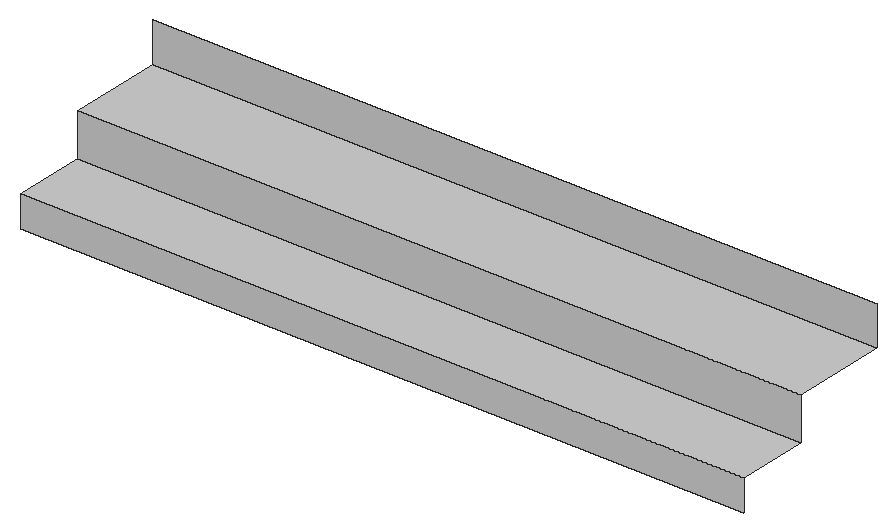
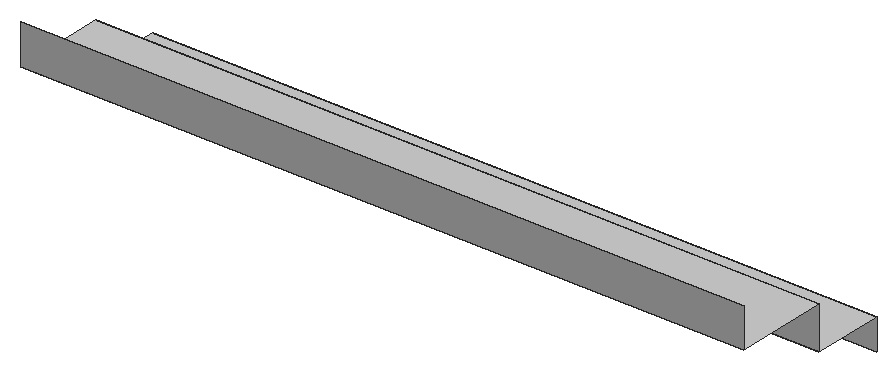
# SketchUp Ruby script. Lengths in inches.
U = 1.inch
M = Sketchup.active_model
def pt(a) = Geom::Point3d.new(a.map { |v| v * U })
def face(e, loops, mat)
  f = e.add_face(loops[0].map { |a| pt(a) })
  loops[1..].each { |l| e.add_face(l.map { |a| pt(a) }).erase! }
  f.material = f.back_material = mat if mat
  f
end
# faces: each face lists its corners as indices into pts; further lists are holes
def faces(e, pts, list, mat = nil) = list.each { |f| face(e, (f[0].is_a?(Array) ? f : [f]).map { |l| l.map { |i| pts[i] } }, mat) }
# xy, xz, yz: faces in a plane at the given z, y or x. An outline is a flat list of corners, or four numbers for a rectangle; further outlines are holes
def ring(l) = l.size == 4 ? [[l[0], l[1]], [l[2], l[1]], [l[2], l[3]], [l[0], l[3]]] : l.each_slice(2).to_a
def flat(e, list, mat, &to3) = list.each { |f| face(e, (f[0].is_a?(Array) ? f : [f]).map { |l| ring(l).map { |u, v| to3.(u, v) } }, mat) }
def xy(e, z, list, mat = nil) = flat(e, list, mat) { |x, y| [x, y, z] }
def xz(e, y, list, mat = nil) = flat(e, list, mat) { |x, z| [x, y, z] }
def yz(e, x, list, mat = nil) = flat(e, list, mat) { |y, z| [x, y, z] }
def lines(e, pts, list) = list.each { |a, b| e.add_line(pt(pts[a]), pt(pts[b])) }
# prism: a flat outline (further loops are holes) pulled along v
def prism(e, loops, v, mat = nil)
  f = face(e, loops, mat); d = Geom::Vector3d.new(v.map { |x| x * U })
  f.pushpull(f.normal.samedirection?(d) ? d.length : -d.length)
end
def box(e, o, s, mat = nil) = prism(e, [[o, [o[0] + s[0], o[1], o[2]], [o[0] + s[0], o[1] + s[1], o[2]], [o[0], o[1] + s[1], o[2]]]], [0, 0, s[2]], mat)
def at(x, y, z, deg = 0) = Geom::Transformation.translation(pt([x, y, z])) * Geom::Transformation.rotation(ORIGIN, Z_AXIS, deg.degrees)
def axes(o, x, y, z) = Geom::Transformation.new([*x, 0, *y, 0, *z, 0, *pt(o).to_a, 1])
def part(name) = M.definitions.add(name)
# library, detail: a bought-in or finely detailed component or shape, given as its bounding box
def library(name, o, s) = part(name).tap { |d| box(d.entities, o, s) }
def detail(e, o, s) = box(e.add_group.entities, o, s)
def put(e, d, t, mat = nil) = e.add_instance(d, t).tap { |i| i.material = mat if mat }
def group(e, t, mat = nil) = e.add_group.tap { |g| g.transformation = t; g.material = mat if mat }.entities
root = M.entities
M.materials.add("[Carrera Marble]").color = [207, 207, 207]
xy(root,28.22,[[111.93,47.98,355.29,71.98]],"[Carrera Marble]")
xy(root,42.68,[[111.93,71.98,355.29,103.86]],"[Carrera Marble]")
xz(root,47.98,[[111.93,17.625,355.29,28.22]],"[Carrera Marble]")
xz(root,71.98,[[111.93,28.22,355.29,42.68]],"[Carrera Marble]")
xz(root,103.86,[[111.93,42.68,355.29,56.07]],"[Carrera Marble]")
